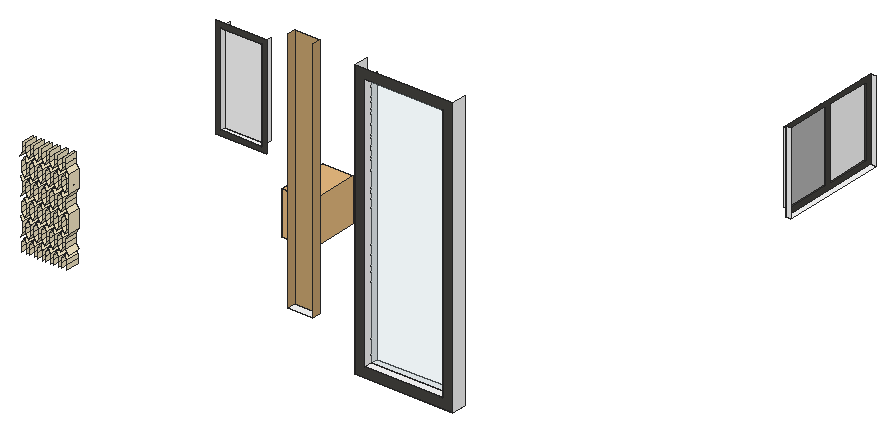
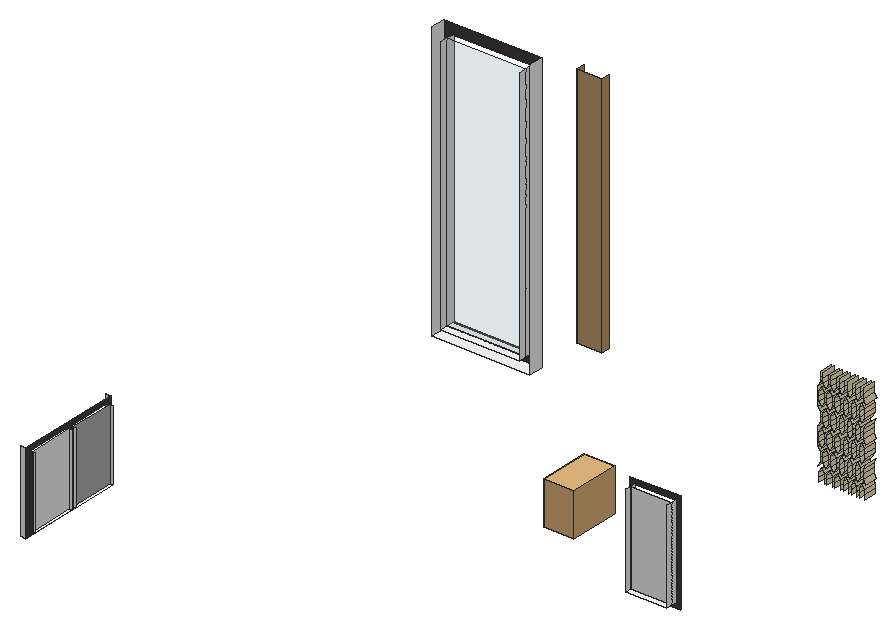
# SketchUp Ruby script. Lengths in inches.
U = 1.inch
M = Sketchup.active_model
def pt(a) = Geom::Point3d.new(a.map { |v| v * U })
def face(e, loops, mat)
  f = e.add_face(loops[0].map { |a| pt(a) })
  loops[1..].each { |l| e.add_face(l.map { |a| pt(a) }).erase! }
  f.material = f.back_material = mat if mat
  f
end
# faces: each face lists its corners as indices into pts; further lists are holes
def faces(e, pts, list, mat = nil) = list.each { |f| face(e, (f[0].is_a?(Array) ? f : [f]).map { |l| l.map { |i| pts[i] } }, mat) }
# xy, xz, yz: faces in a plane at the given z, y or x. An outline is a flat list of corners, or four numbers for a rectangle; further outlines are holes
def ring(l) = l.size == 4 ? [[l[0], l[1]], [l[2], l[1]], [l[2], l[3]], [l[0], l[3]]] : l.each_slice(2).to_a
def flat(e, list, mat, &to3) = list.each { |f| face(e, (f[0].is_a?(Array) ? f : [f]).map { |l| ring(l).map { |u, v| to3.(u, v) } }, mat) }
def xy(e, z, list, mat = nil) = flat(e, list, mat) { |x, y| [x, y, z] }
def xz(e, y, list, mat = nil) = flat(e, list, mat) { |x, z| [x, y, z] }
def yz(e, x, list, mat = nil) = flat(e, list, mat) { |y, z| [x, y, z] }
def lines(e, pts, list) = list.each { |a, b| e.add_line(pt(pts[a]), pt(pts[b])) }
# prism: a flat outline (further loops are holes) pulled along v
def prism(e, loops, v, mat = nil)
  f = face(e, loops, mat); d = Geom::Vector3d.new(v.map { |x| x * U })
  f.pushpull(f.normal.samedirection?(d) ? d.length : -d.length)
end
def box(e, o, s, mat = nil) = prism(e, [[o, [o[0] + s[0], o[1], o[2]], [o[0] + s[0], o[1] + s[1], o[2]], [o[0], o[1] + s[1], o[2]]]], [0, 0, s[2]], mat)
def at(x, y, z, deg = 0) = Geom::Transformation.translation(pt([x, y, z])) * Geom::Transformation.rotation(ORIGIN, Z_AXIS, deg.degrees)
def axes(o, x, y, z) = Geom::Transformation.new([*x, 0, *y, 0, *z, 0, *pt(o).to_a, 1])
def part(name) = M.definitions.add(name)
# library, detail: a bought-in or finely detailed component or shape, given as its bounding box
def library(name, o, s) = part(name).tap { |d| box(d.entities, o, s) }
def detail(e, o, s) = box(e.add_group.entities, o, s)
def put(e, d, t, mat = nil) = e.add_instance(d, t).tap { |i| i.material = mat if mat }
def group(e, t, mat = nil) = e.add_group.tap { |g| g.transformation = t; g.material = mat if mat }.entities
root = M.entities
M.materials.add("D01_Frost_White").color = [255, 242, 206]
M.materials.add("Glass_Mirror_01").color = [185, 185, 185]
M.materials.add("Glass_Safety_01").color = [204, 235, 244]
M.materials["Glass_Safety_01"].alpha = 0.25
M.materials.add("M00_Soft_Cloud").color = [255, 255, 255]
M.materials.add("Plywood_08_1K").color = [202, 166, 113]
M.materials.add("Wood_Planks_01_1K").color = [69, 67, 63]
c1 = library("FF_Model_ID8636_1_ruthrocker1",[-22.29,-12.06,-2.32],[42.44,25.59,36.01])
xy(root,142.2252,[[455.5996,116.0568,536.8247,128.0311]],"M00_Soft_Cloud")
xy(root,145.482,[[189.7692,309,223.7462,313.5],[189.7692,313.5,223.7462,318]],"M00_Soft_Cloud")
xy(root,150.2252,[[463.5996,116.0568,528.8247,122.5284],[463.5996,122.5284,528.8247,129]],"M00_Soft_Cloud")
xy(root,156.7042,[[559.3018,433.068,564,521.5592]],"M00_Soft_Cloud")
xy(root,160.7042,[[555,437.068,557.1509,475.3136],[555,479.3136,557.1509,517.5592]],"M00_Soft_Cloud")
xy(root,160.7042,[[557.1509,437.068,559.3018,475.3136],[557.1509,479.3136,559.3018,517.5592]],"Wood_Planks_01_1K")
xy(root,173.8079,[[402.037,112.9098,423.1418,120]],"M00_Soft_Cloud")
xy(root,197.0101,[[189.8495,109.0676,189.8566,119.6039],[196.5404,109.0676,196.5475,119.6039],[209.9258,109.0676,209.9294,119.6039],[216.6168,109.0676,216.6239,119.6039],[223.3077,109.0676,223.3148,119.6039]],"D01_Frost_White")
xy(root,197.0162,[[189.853,109.0676,189.8602,119.6039],[196.544,109.0676,196.5511,119.6039]],"D01_Frost_White")
xz(root,109.0676,[[216.6203,197.004,216.6239,197.0101,216.6168,197.0101,216.6184,197.0073],[209.9276,197.0071,209.9294,197.0101,209.9258,197.0101],[189.8495,197.0101,189.8566,197.0101,189.8547,197.0134,189.853,197.0162,189.8514,197.0134],[189.8566,197.0101,189.8602,197.0162,189.853,197.0162,189.8547,197.0134],[189.8566,197.0101,189.8637,197.0101,189.8602,197.0162],
  [196.5404,197.0101,196.5475,197.0101,196.5511,197.0162,196.544,197.0162],[196.5475,197.0101,196.5547,197.0101,196.5546,197.0102,196.5511,197.0162],[203.2385,197.0101,203.2456,197.0101,203.2437,197.0134,203.242,197.0162,203.2404,197.0134],[209.933,212.0139,209.933,212.02,209.9312,212.0169]],"D01_Frost_White")
xz(root,116.0568,[[[455.5996,142.2252,536.8247,372.3605],[463.5996,150.2252,528.8247,364.3605]]],"Wood_Planks_01_1K")
xz(root,120,[[402.037,173.8079,423.1418,377.6765]],"Plywood_08_1K")
xz(root,122.5284,[[463.5996,150.2252,528.8247,364.3605]],"Glass_Safety_01")
xz(root,309,[[[185.7692,141.482,227.7462,225.934],[189.7692,145.482,223.7462,221.934]]],"Wood_Planks_01_1K")
xz(root,313.5,[[189.7692,145.482,223.7462,221.934]],"M00_Soft_Cloud")
xz(root,433.068,[[559.3018,156.7042,564,224.1287]],"M00_Soft_Cloud")
xz(root,437.068,[[555,160.7042,557.1509,220.1287]],"M00_Soft_Cloud")
xz(root,437.068,[[557.1509,160.7042,559.3018,220.1287]],"Wood_Planks_01_1K")
xz(root,475.3136,[[555,160.7042,557.1509,220.1287]],"M00_Soft_Cloud")
xz(root,475.3136,[[557.1509,160.7042,559.3018,220.1287]],"Wood_Planks_01_1K")
xz(root,479.3136,[[555,160.7042,557.1509,220.1287],[557.1509,160.7042,559.3018,220.1287]],"M00_Soft_Cloud")
xz(root,517.5592,[[555,160.7042,557.1509,220.1287]],"M00_Soft_Cloud")
xz(root,517.5592,[[557.1509,160.7042,559.3018,220.1287]],"Wood_Planks_01_1K")
xz(root,521.5592,[[559.3018,156.7042,564,224.1287]],"M00_Soft_Cloud")
yz(root,184.3035,[[109.0676,200.7656,119.6039,204.515],[109.0676,204.515,119.6039,208.2645]],"D01_Frost_White")
yz(root,184.3107,[[109.0676,140.7747,119.6039,144.5242],[109.0676,144.5242,119.6039,148.2736],[109.0676,170.7702,119.6039,174.5196],[109.0676,174.5196,119.6039,178.269]],"D01_Frost_White")
yz(root,185.3661,[[109.0676,215.7633,119.6039,219.5128],[109.0676,219.5128,119.6039,223.2622]],"D01_Frost_White")
yz(root,185.3733,[[109.0676,155.7725,119.6039,159.5219],[109.0676,159.5219,119.6039,163.2713],[109.0676,185.7679,119.6039,189.5173],[109.0676,189.5173,119.6039,193.2668]],"D01_Frost_White")
yz(root,187.649,[[109.0676,215.7633,119.6039,219.5128],[109.0676,219.5128,119.6039,223.2622]],"D01_Frost_White")
yz(root,187.6561,[[109.0676,155.7725,119.6039,159.5219],[109.0676,159.5219,119.6039,163.2713],[109.0676,185.7679,119.6039,189.5173],[109.0676,189.5173,119.6039,193.2668]],"D01_Frost_White")
yz(root,188.7116,[[109.0676,200.7656,119.6039,204.515],[109.0676,204.515,119.6039,208.2645]],"D01_Frost_White")
yz(root,188.7188,[[109.0676,140.7747,119.6039,144.5242],[109.0676,144.5242,119.6039,148.2736],[109.0676,170.7702,119.6039,174.5196],[109.0676,174.5196,119.6039,178.269]],"D01_Frost_White")
yz(root,189.7692,[[309,145.482,313.5,221.934],[313.5,145.482,318,221.934]],"M00_Soft_Cloud")
yz(root,190.9945,[[109.0676,200.7656,119.6039,204.515],[109.0676,204.515,119.6039,208.2645]],"D01_Frost_White")
yz(root,191.0016,[[109.0676,140.7747,119.6039,144.5242],[109.0676,144.5242,119.6039,148.2736],[109.0676,170.7702,119.6039,174.5196],[109.0676,174.5196,119.6039,178.269]],"D01_Frost_White")
yz(root,192.0571,[[109.0676,215.7633,119.6039,219.5128],[109.0676,219.5128,119.6039,223.2622]],"D01_Frost_White")
yz(root,192.0642,[[109.0676,155.7725,119.6039,159.5219],[109.0676,159.5219,119.6039,163.2713],[109.0676,185.7679,119.6039,189.5173],[109.0676,189.5173,119.6039,193.2668]],"D01_Frost_White")
yz(root,194.3399,[[109.0676,215.7633,119.6039,219.5128],[109.0676,219.5128,119.6039,223.2622]],"D01_Frost_White")
yz(root,194.3471,[[109.0676,155.7725,119.6039,159.5219],[109.0676,159.5219,119.6039,163.2713],[109.0676,185.7679,119.6039,189.5173],[109.0676,189.5173,119.6039,193.2668]],"D01_Frost_White")
yz(root,195.4025,[[109.0676,200.7656,119.6039,204.515],[109.0676,204.515,119.6039,208.2645]],"D01_Frost_White")
yz(root,195.4097,[[109.0676,140.7747,119.6039,144.5242],[109.0676,144.5242,119.6039,148.2736],[109.0676,170.7702,119.6039,174.5196],[109.0676,174.5196,119.6039,178.269]],"D01_Frost_White")
yz(root,197.6925,[[109.0676,140.7747,119.6039,144.5242],[109.0676,144.5242,119.6039,148.2736],[109.0676,170.7702,119.6039,174.5196],[109.0676,174.5196,119.6039,178.269],[109.0676,200.7656,119.6039,204.515],
  [109.0676,204.515,119.6039,208.2645]],"D01_Frost_White")
yz(root,198.748,[[109.0676,215.7633,119.6039,223.2622]],"D01_Frost_White")
yz(root,198.7552,[[109.0676,155.7725,119.6039,159.5219],[109.0676,159.5219,119.6039,163.2713],[109.0676,185.7679,119.6039,189.5173],[109.0676,189.5173,119.6039,193.2668]],"D01_Frost_White")
yz(root,201.038,[[109.0676,155.7725,119.6039,159.5219],[109.0676,159.5219,119.6039,163.2713],[109.0676,185.7679,119.6039,189.5173],[109.0676,189.5173,119.6039,193.2668],[109.0676,215.7633,119.6039,219.5128],
  [109.0676,219.5128,119.6039,223.2622]],"D01_Frost_White")
yz(root,202.1006,[[109.0676,140.7747,119.6039,144.5242],[109.0676,144.5242,119.6039,148.2736],[109.0676,170.7702,119.6039,174.5196],[109.0676,174.5196,119.6039,178.269],[109.0676,200.7656,119.6039,204.515],
  [109.0676,204.515,119.6039,208.2645]],"D01_Frost_White")
yz(root,204.3835,[[109.0676,140.7747,119.6039,144.5242],[109.0676,144.5242,119.6039,148.2736],[109.0676,170.7702,119.6039,174.5196],[109.0676,174.5196,119.6039,178.269],[109.0676,200.7656,119.6039,204.515],
  [109.0676,204.515,119.6039,208.2645]],"D01_Frost_White")
yz(root,205.4461,[[109.0676,155.7725,119.6039,159.5219],[109.0676,159.5219,119.6039,163.2713],[109.0676,185.7679,119.6039,189.5173],[109.0676,189.5173,119.6039,193.2668],[109.0676,215.7633,119.6039,219.5128],
  [109.0676,219.5128,119.6039,223.2622]],"D01_Frost_White")
yz(root,207.7289,[[109.0676,155.7725,119.6039,159.5219],[109.0676,159.5219,119.6039,163.2713],[109.0676,185.7679,119.6039,189.5173],[109.0676,189.5173,119.6039,193.2668],[109.0676,215.7633,119.6039,219.5128],
  [109.0676,219.5128,119.6039,223.2622]],"D01_Frost_White")
yz(root,208.7916,[[109.0676,140.7747,119.6039,144.5242],[109.0676,144.5242,119.6039,148.2736],[109.0676,170.7702,119.6039,174.5196],[109.0676,174.5196,119.6039,178.269],[109.0676,200.7656,119.6039,204.515],
  [109.0676,204.515,119.6039,208.2645]],"D01_Frost_White")
yz(root,209.933,[[109.0676,152.0169,119.6039,152.023],[109.0676,167.0147,119.6039,167.0207],[109.0676,182.0124,119.6039,182.0185],[109.0676,197.0101,119.6039,197.0162],[109.0676,212.0139,119.6039,212.02]],"D01_Frost_White")
yz(root,211.0673,[[109.0676,200.7595,119.6039,204.509],[109.0676,204.509,119.6039,208.2584]],"D01_Frost_White")
yz(root,211.0744,[[109.0676,140.7687,119.6039,144.5181],[109.0676,144.5181,119.6039,148.2675],[109.0676,170.7641,119.6039,174.5135],[109.0676,174.5135,119.6039,178.263]],"D01_Frost_White")
yz(root,212.1299,[[109.0676,215.7573,119.6039,219.5067],[109.0676,219.5067,119.6039,223.2561]],"D01_Frost_White")
yz(root,212.137,[[109.0676,155.7664,119.6039,159.5158],[109.0676,159.5158,119.6039,163.2652],[109.0676,185.7618,119.6039,189.5113],[109.0676,189.5113,119.6039,193.2607]],"D01_Frost_White")
yz(root,214.4127,[[109.0676,215.7573,119.6039,219.5067],[109.0676,219.5067,119.6039,223.2561]],"D01_Frost_White")
yz(root,214.4199,[[109.0676,155.7664,119.6039,159.5158],[109.0676,159.5158,119.6039,163.2652],[109.0676,185.7618,119.6039,189.5113],[109.0676,189.5113,119.6039,193.2607]],"D01_Frost_White")
yz(root,215.4754,[[109.0676,200.7595,119.6039,204.509],[109.0676,204.509,119.6039,208.2584]],"D01_Frost_White")
yz(root,215.4825,[[109.0676,140.7687,119.6039,144.5181],[109.0676,144.5181,119.6039,148.2675],[109.0676,170.7641,119.6039,174.5135],[109.0676,174.5135,119.6039,178.263]],"D01_Frost_White")
yz(root,217.7582,[[109.0676,200.7595,119.6039,204.509],[109.0676,204.509,119.6039,208.2584]],"D01_Frost_White")
yz(root,217.7653,[[109.0676,140.7687,119.6039,144.5181],[109.0676,144.5181,119.6039,148.2675],[109.0676,170.7641,119.6039,174.5135],[109.0676,174.5135,119.6039,178.263]],"D01_Frost_White")
yz(root,218.8208,[[109.0676,215.7573,119.6039,219.5067],[109.0676,219.5067,119.6039,223.2561]],"D01_Frost_White")
yz(root,218.828,[[109.0676,155.7664,119.6039,159.5158],[109.0676,159.5158,119.6039,163.2652],[109.0676,185.7618,119.6039,189.5113],[109.0676,189.5113,119.6039,193.2607]],"D01_Frost_White")
yz(root,221.1037,[[109.0676,215.7573,119.6039,219.5067],[109.0676,219.5067,119.6039,223.2561]],"D01_Frost_White")
yz(root,221.1108,[[109.0676,155.7664,119.6039,159.5158],[109.0676,159.5158,119.6039,163.2652],[109.0676,185.7618,119.6039,189.5113],[109.0676,189.5113,119.6039,193.2607]],"D01_Frost_White")
yz(root,222.1663,[[109.0676,200.7595,119.6039,204.509],[109.0676,204.509,119.6039,208.2584]],"D01_Frost_White")
yz(root,222.1734,[[109.0676,140.7687,119.6039,144.5181],[109.0676,144.5181,119.6039,148.2675],[109.0676,170.7641,119.6039,174.5135],[109.0676,174.5135,119.6039,178.263]],"D01_Frost_White")
yz(root,223.3077,[[109.0676,197.0101,119.6039,212.0078]],"D01_Frost_White")
yz(root,223.3148,[[109.0676,167.0147,119.6039,182.0124]],"D01_Frost_White")
yz(root,223.7462,[[309,145.482,313.5,221.934],[313.5,145.482,318,221.934]],"M00_Soft_Cloud")
yz(root,402.037,[[112.9098,173.8079,120,377.6765]],"Plywood_08_1K")
yz(root,423.1418,[[112.9098,173.8079,120,377.6765]],"Plywood_08_1K")
yz(root,455.5996,[[116.0568,142.2252,128.0311,372.3605]],"M00_Soft_Cloud")
yz(root,463.5996,[[116.0568,150.2252,122.5284,364.3605],[122.5284,150.2252,129,364.3605]],"M00_Soft_Cloud")
yz(root,528.8247,[[116.0568,150.2252,122.5284,364.3605],[122.5284,150.2252,129,364.3605]],"M00_Soft_Cloud")
yz(root,536.8247,[[116.0568,142.2252,128.0311,372.3605]],"M00_Soft_Cloud")
yz(root,557.1509,[[437.068,160.7042,475.3136,220.1287]],"Glass_Mirror_01")
yz(root,557.1509,[[479.3136,160.7042,517.5592,220.1287]],"M00_Soft_Cloud")
yz(root,559.3018,[[[433.068,156.7042,521.5592,224.1287],[437.068,160.7042,475.3136,220.1287],[479.3136,160.7042,517.5592,220.1287]]],"Wood_Planks_01_1K")
p = [[184.3107,109.0676,148.2736],[186.5147,109.0676,152.023],[186.5147,119.6039,152.023],[184.3107,119.6039,148.2736],[188.7188,109.0676,148.2736],[188.7188,119.6039,148.2736],
  [191.0016,109.0676,148.2736],[193.2056,109.0676,152.023],[193.2056,119.6039,152.023],[191.0016,119.6039,148.2736],[195.4097,109.0676,148.2736],[195.4097,119.6039,148.2736],
  [197.6925,109.0676,148.2736],[199.8966,109.0676,152.023],[199.8966,119.6039,152.023],[197.6925,119.6039,148.2736],[202.1006,109.0676,148.2736],[202.1006,119.6039,148.2736],
  [204.3835,109.0676,148.2736],[206.5875,109.0676,152.023],[206.5875,119.6039,152.023],[204.3835,119.6039,148.2736],[208.7916,109.0676,148.2736],[208.7916,119.6039,148.2736],
  [211.0744,109.0676,148.2675],[213.2784,109.0676,152.0169],[213.2784,119.6039,152.0169],[211.0744,119.6039,148.2675],[215.4825,109.0676,148.2675],[215.4825,119.6039,148.2675],
  [217.7653,109.0676,148.2675],[219.9694,109.0676,152.0169],[219.9694,119.6039,152.0169],[217.7653,119.6039,148.2675],[222.1734,109.0676,148.2675],[222.1734,119.6039,148.2675],
  [185.3733,109.0676,155.7725],[183.1692,109.0676,152.023],[183.1692,119.6039,152.023],[185.3733,119.6039,155.7725],[189.8602,109.0676,152.023],[187.6561,109.0676,155.7725],
  [187.6561,119.6039,155.7725],[189.8602,119.6039,152.023],[192.0642,109.0676,155.7725],[192.0642,119.6039,155.7725],[196.5511,109.0676,152.023],[194.3471,109.0676,155.7725],
  [194.3471,119.6039,155.7725],[196.5511,119.6039,152.023],[198.7552,109.0676,155.7725],[198.7552,119.6039,155.7725],[203.242,109.0676,152.023],[201.038,109.0676,155.7725],
  [201.038,119.6039,155.7725],[203.242,119.6039,152.023],[205.4461,109.0676,155.7725],[205.4461,119.6039,155.7725],[209.933,109.0676,152.023],[207.7289,109.0676,155.7725],
  [207.7289,119.6039,155.7725],[209.933,119.6039,152.023],[212.137,109.0676,155.7664],[209.933,109.0676,152.0169],[209.933,119.6039,152.0169],[212.137,119.6039,155.7664],
  [216.6239,109.0676,152.0169],[214.4199,109.0676,155.7664],[214.4199,119.6039,155.7664],[216.6239,119.6039,152.0169],[218.828,109.0676,155.7664],[218.828,119.6039,155.7664],
  [223.3148,109.0676,152.0169],[221.1108,109.0676,155.7664],[221.1108,119.6039,155.7664],[223.3148,119.6039,152.0169],[183.1692,109.0676,167.0207],[185.3733,109.0676,163.2713],
  [185.3733,119.6039,163.2713],[183.1692,119.6039,167.0207],[187.6561,109.0676,163.2713],[189.8602,109.0676,167.0207],[189.8602,119.6039,167.0207],[187.6561,119.6039,163.2713],
  [192.0642,109.0676,163.2713],[192.0642,119.6039,163.2713],[194.3471,109.0676,163.2713],[196.5511,109.0676,167.0207],[196.5511,119.6039,167.0207],[194.3471,119.6039,163.2713],
  [198.7552,109.0676,163.2713],[198.7552,119.6039,163.2713],[201.038,109.0676,163.2713],[203.242,109.0676,167.0207],[203.242,119.6039,167.0207],[201.038,119.6039,163.2713],
  [205.4461,109.0676,163.2713],[205.4461,119.6039,163.2713],[207.7289,109.0676,163.2713],[209.933,109.0676,167.0207],[209.933,119.6039,167.0207],[207.7289,119.6039,163.2713],
  [209.933,109.0676,167.0147],[212.137,109.0676,163.2652],[212.137,119.6039,163.2652],[209.933,119.6039,167.0147],[214.4199,109.0676,163.2652],[216.6239,109.0676,167.0147],
  [216.6239,119.6039,167.0147],[214.4199,119.6039,163.2652],[218.828,109.0676,163.2652],[218.828,119.6039,163.2652],[221.1108,109.0676,163.2652],[223.3148,109.0676,167.0147],
  [223.3148,119.6039,167.0147],[221.1108,119.6039,163.2652],[186.5147,109.0676,167.0207],[184.3107,109.0676,170.7702],[184.3107,119.6039,170.7702],[186.5147,119.6039,167.0207],
  [188.7188,109.0676,170.7702],[188.7188,119.6039,170.7702],[193.2056,109.0676,167.0207],[191.0016,109.0676,170.7702],[191.0016,119.6039,170.7702],[193.2056,119.6039,167.0207],
  [195.4097,109.0676,170.7702],[195.4097,119.6039,170.7702],[199.8966,109.0676,167.0207],[197.6925,109.0676,170.7702],[197.6925,119.6039,170.7702],[199.8966,119.6039,167.0207],
  [202.1006,109.0676,170.7702],[202.1006,119.6039,170.7702],[206.5875,109.0676,167.0207],[204.3835,109.0676,170.7702],[204.3835,119.6039,170.7702],[206.5875,119.6039,167.0207],
  [208.7916,109.0676,170.7702],[208.7916,119.6039,170.7702],[213.2784,109.0676,167.0147],[211.0744,109.0676,170.7641],[211.0744,119.6039,170.7641],[213.2784,119.6039,167.0147],
  [215.4825,109.0676,170.7641],[215.4825,119.6039,170.7641],[219.9694,109.0676,167.0147],[217.7653,109.0676,170.7641],[217.7653,119.6039,170.7641],[219.9694,119.6039,167.0147],
  [222.1734,109.0676,170.7641],[222.1734,119.6039,170.7641],[184.3107,109.0676,178.269],[186.5147,109.0676,182.0185],[186.5147,119.6039,182.0185],[184.3107,119.6039,178.269],
  [188.7188,109.0676,178.269],[188.7188,119.6039,178.269],[191.0016,109.0676,178.269],[193.2056,109.0676,182.0185],[193.2056,119.6039,182.0185],[191.0016,119.6039,178.269],
  [195.4097,109.0676,178.269],[195.4097,119.6039,178.269],[197.6925,109.0676,178.269],[199.8966,109.0676,182.0185],[199.8966,119.6039,182.0185],[197.6925,119.6039,178.269],
  [202.1006,109.0676,178.269],[202.1006,119.6039,178.269],[204.3835,109.0676,178.269],[206.5875,109.0676,182.0185],[206.5875,119.6039,182.0185],[204.3835,119.6039,178.269],
  [208.7916,109.0676,178.269],[208.7916,119.6039,178.269],[211.0744,109.0676,178.263],[213.2784,109.0676,182.0124],[213.2784,119.6039,182.0124],[211.0744,119.6039,178.263],
  [215.4825,109.0676,178.263],[215.4825,119.6039,178.263],[217.7653,109.0676,178.263],[219.9694,109.0676,182.0124],[219.9694,119.6039,182.0124],[217.7653,119.6039,178.263],
  [222.1734,109.0676,178.263],[222.1734,119.6039,178.263],[185.3733,109.0676,185.7679],[183.1692,109.0676,182.0185],[183.1692,119.6039,182.0185],[185.3733,119.6039,185.7679],
  [189.8602,109.0676,182.0185],[187.6561,109.0676,185.7679],[187.6561,119.6039,185.7679],[189.8602,119.6039,182.0185],[192.0642,109.0676,185.7679],[192.0642,119.6039,185.7679],
  [196.5511,109.0676,182.0185],[194.3471,109.0676,185.7679],[194.3471,119.6039,185.7679],[196.5511,119.6039,182.0185],[198.7552,109.0676,185.7679],[198.7552,119.6039,185.7679],
  [203.242,109.0676,182.0185],[201.038,109.0676,185.7679],[201.038,119.6039,185.7679],[203.242,119.6039,182.0185],[205.4461,109.0676,185.7679],[205.4461,119.6039,185.7679],
  [209.933,109.0676,182.0185],[207.7289,109.0676,185.7679],[207.7289,119.6039,185.7679],[209.933,119.6039,182.0185],[212.137,109.0676,185.7618],[209.933,109.0676,182.0124],
  [209.933,119.6039,182.0124],[212.137,119.6039,185.7618],[216.6239,109.0676,182.0124],[214.4199,109.0676,185.7618],[214.4199,119.6039,185.7618],[216.6239,119.6039,182.0124],
  [218.828,109.0676,185.7618],[218.828,119.6039,185.7618],[223.3148,109.0676,182.0124],[221.1108,109.0676,185.7618],[221.1108,119.6039,185.7618],[223.3148,119.6039,182.0124],
  [183.1728,109.0676,197.0101],[185.3733,109.0676,193.2668],[185.3733,119.6039,193.2668],[183.1728,119.6039,197.0101],[187.6561,109.0676,193.2668],[189.8566,109.0676,197.0101],
  [189.8566,119.6039,197.0101],[187.6561,119.6039,193.2668],[189.8637,109.0676,197.0101],[192.0642,109.0676,193.2668],[192.0642,119.6039,193.2668],[189.8637,119.6039,197.0101],
  [194.3471,109.0676,193.2668],[196.5475,109.0676,197.0101],[196.5475,119.6039,197.0101],[194.3471,119.6039,193.2668],[196.5547,109.0676,197.0101],[198.7552,109.0676,193.2668],
  [198.7552,119.6039,193.2668],[196.5547,119.6039,197.0101],[201.038,109.0676,193.2668],[203.2385,109.0676,197.0101],[203.2385,119.6039,197.0101],[201.038,119.6039,193.2668],
  [203.2456,109.0676,197.0101],[205.4461,109.0676,193.2668],[205.4461,119.6039,193.2668],[203.2456,119.6039,197.0101],[207.7289,109.0676,193.2668],[209.9276,109.0676,197.0071],
  [209.9276,119.6039,197.0071],[207.7289,119.6039,193.2668],[209.933,109.0676,197.0101],[212.137,109.0676,193.2607],[212.137,119.6039,193.2607],[209.933,119.6039,197.0101],
  [214.4199,109.0676,193.2607],[216.6203,109.0676,197.004],[216.6203,119.6039,197.004],[214.4199,119.6039,193.2607],[216.6239,109.0676,197.0101],[218.828,109.0676,193.2607],
  [218.828,119.6039,193.2607],[216.6239,119.6039,197.0101],[221.1108,109.0676,193.2607],[223.3148,109.0676,197.0101],[223.3148,119.6039,197.0101],[221.1108,119.6039,193.2607],
  [186.5076,109.0676,197.0162],[184.3035,109.0676,200.7656],[184.3035,119.6039,200.7656],[186.5076,119.6039,197.0162],[188.7116,109.0676,200.7656],[188.7116,119.6039,200.7656],
  [189.8495,109.0676,197.0101],[189.8514,109.0676,197.0134],[189.8514,119.6039,197.0134],[189.8495,119.6039,197.0101],[189.853,109.0676,197.0162],[189.853,119.6039,197.0162],
  [189.8602,109.0676,197.0162],[189.8602,119.6039,197.0162],[193.1985,109.0676,197.0162],[190.9945,109.0676,200.7656],[190.9945,119.6039,200.7656],[193.1985,119.6039,197.0162],
  [195.4025,109.0676,200.7656],[195.4025,119.6039,200.7656],[196.5404,109.0676,197.0101],[196.544,109.0676,197.0162],[196.544,119.6039,197.0162],[196.5404,119.6039,197.0101],
  [196.5511,109.0676,197.0162],[196.5546,109.0676,197.0102],[196.5546,119.6039,197.0102],[196.5511,119.6039,197.0162],[199.8966,109.0676,197.0162],[197.6925,109.0676,200.7656],
  [197.6925,119.6039,200.7656],[199.8966,119.6039,197.0162],[202.1006,109.0676,200.7656],[202.1006,119.6039,200.7656],[203.2404,109.0676,197.0134],[203.2404,119.6039,197.0134],
  [203.242,109.0676,197.0162],[203.242,119.6039,197.0162],[203.2437,109.0676,197.0134],[203.2437,119.6039,197.0134],[206.5875,109.0676,197.0162],[204.3835,109.0676,200.7656],
  [204.3835,119.6039,200.7656],[206.5875,119.6039,197.0162],[208.7916,109.0676,200.7656],[208.7916,119.6039,200.7656],[209.9258,109.0676,197.0101],[209.9258,119.6039,197.0101],
  [209.9294,109.0676,197.0101],[209.933,109.0676,197.0162],[209.933,119.6039,197.0162],[209.9294,119.6039,197.0101],[213.2713,109.0676,197.0101],[211.0673,109.0676,200.7595],
  [211.0673,119.6039,200.7595],[213.2713,119.6039,197.0101],[215.4754,109.0676,200.7595],[215.4754,119.6039,200.7595],[216.6184,109.0676,197.0073],[216.6168,109.0676,197.0101],
  [216.6168,119.6039,197.0101],[216.6184,119.6039,197.0073],[219.9622,109.0676,197.0101],[217.7582,109.0676,200.7595],[217.7582,119.6039,200.7595],[219.9622,119.6039,197.0101],
  [222.1663,109.0676,200.7595],[222.1663,119.6039,200.7595],[184.3035,109.0676,208.2645],[186.5076,109.0676,212.0139],[186.5076,119.6039,212.0139],[184.3035,119.6039,208.2645],
  [188.7116,109.0676,208.2645],[188.7116,119.6039,208.2645],[190.9945,109.0676,208.2645],[193.1985,109.0676,212.0139],[193.1985,119.6039,212.0139],[190.9945,119.6039,208.2645],
  [195.4025,109.0676,208.2645],[195.4025,119.6039,208.2645],[197.6925,109.0676,208.2645],[199.8966,109.0676,212.0139],[199.8966,119.6039,212.0139],[197.6925,119.6039,208.2645],
  [202.1006,109.0676,208.2645],[202.1006,119.6039,208.2645],[204.3835,109.0676,208.2645],[206.5875,109.0676,212.0139],[206.5875,119.6039,212.0139],[204.3835,119.6039,208.2645],
  [208.7916,109.0676,208.2645],[208.7916,119.6039,208.2645],[211.0673,109.0676,208.2584],[213.2713,109.0676,212.0078],[213.2713,119.6039,212.0078],[211.0673,119.6039,208.2584],
  [215.4754,109.0676,208.2584],[215.4754,119.6039,208.2584],[217.7582,109.0676,208.2584],[219.9622,109.0676,212.0078],[219.9622,119.6039,212.0078],[217.7582,119.6039,208.2584],
  [222.1663,109.0676,208.2584],[222.1663,119.6039,208.2584],[185.3661,109.0676,215.7633],[183.1675,109.0676,212.023],[183.1675,119.6039,212.023],[185.3661,119.6039,215.7633],
  [189.853,109.0676,212.0139],[187.649,109.0676,215.7633],[187.649,119.6039,215.7633],[189.853,119.6039,212.0139],[192.0571,109.0676,215.7633],[192.0571,119.6039,215.7633],
  [196.544,109.0676,212.0139],[194.3399,109.0676,215.7633],[194.3399,119.6039,215.7633],[196.544,119.6039,212.0139],[198.748,109.0676,215.7633],[198.748,119.6039,215.7633],
  [203.242,109.0676,212.0139],[201.038,109.0676,215.7633],[201.038,119.6039,215.7633],[203.242,119.6039,212.0139],[205.4461,109.0676,215.7633],[205.4461,119.6039,215.7633],
  [209.9312,109.0676,212.0169],[207.7289,109.0676,215.7633],[207.7289,119.6039,215.7633],[209.9312,119.6039,212.0169],[209.933,109.0676,212.0139],[209.933,119.6039,212.0139],
  [212.1299,109.0676,215.7573],[209.933,109.0676,212.02],[209.933,119.6039,212.02],[212.1299,119.6039,215.7573],[216.6168,109.0676,212.0078],[214.4127,109.0676,215.7573],
  [214.4127,119.6039,215.7573],[216.6168,119.6039,212.0078],[218.8208,109.0676,215.7573],[218.8208,119.6039,215.7573],[223.3077,109.0676,212.0078],[221.1037,109.0676,215.7573],
  [221.1037,119.6039,215.7573],[223.3077,119.6039,212.0078],[209.9276,109.0676,212.0109],[223.3041,109.0676,197.004],[223.3077,109.0676,197.0101],[209.9294,109.0676,197.0041],
  [209.9258,109.0676,212.0078],[209.9294,109.0676,197.004],[216.6151,109.0676,197.0074],[216.6132,109.0676,197.004]]
faces(root,p,[[0,1,2,3],[1,4,5,2],[6,7,8,9],[7,10,11,8],[12,13,14,15],[13,16,17,14],[18,19,20,21],[19,22,23,20],
  [24,25,26,27],[25,28,29,26],[30,31,32,33],[31,34,35,32],[36,37,38,39],[40,41,42,43],[44,40,43,45],[46,47,48,49],
  [50,46,49,51],[52,53,54,55],[56,52,55,57],[58,59,60,61],[62,63,64,65],[66,67,68,69],[70,66,69,71],[72,73,74,75],
  [76,77,78,79],[80,81,82,83],[81,84,85,82],[86,87,88,89],[87,90,91,88],[92,93,94,95],[93,96,97,94],[98,99,100,101],
  [102,103,104,105],[106,107,108,109],[107,110,111,108],[112,113,114,115],[116,117,118,119],[120,116,119,121],[122,123,124,125],[126,122,125,127],
  [128,129,130,131],[132,128,131,133],[134,135,136,137],[138,134,137,139],[140,141,142,143],[144,140,143,145],[146,147,148,149],[150,146,149,151],
  [152,153,154,155],[153,156,157,154],[158,159,160,161],[159,162,163,160],[164,165,166,167],[165,168,169,166],[170,171,172,173],[171,174,175,172],
  [176,177,178,179],[177,180,181,178],[182,183,184,185],[183,186,187,184],[188,189,190,191],[192,193,194,195],[196,192,195,197],[198,199,200,201],
  [202,198,201,203],[204,205,206,207],[208,204,207,209],[210,211,212,213],[214,215,216,217],[218,219,220,221],[222,218,221,223],[224,225,226,227],
  [228,229,230,231],[232,233,234,235],[236,237,238,239],[240,241,242,243],[244,245,246,247],[248,249,250,251],[252,253,254,255],[256,257,258,259],
  [260,261,262,263],[264,265,266,267],[268,269,270,271],[272,273,274,275],[276,277,278,279],[280,276,279,281],[282,283,284,285],[283,286,287,284],
  [288,236,239,289],[290,291,292,293],[294,290,293,295],[296,297,298,299],[300,301,302,303],[301,244,247,302],[304,305,306,307],[308,304,307,309],
  [249,310,311,250],[310,312,313,311],[312,314,315,313],[314,252,255,315],[316,317,318,319],[320,316,319,321],[257,322,323,258],[324,325,326,327],
  [328,329,330,331],[332,328,331,333],[334,335,336,337],[265,334,337,266],[338,339,340,341],[342,338,341,343],[344,345,346,347],[345,348,349,346],
  [350,351,352,353],[351,354,355,352],[356,357,358,359],[357,360,361,358],[362,363,364,365],[363,366,367,364],[368,369,370,371],[369,372,373,370],
  [374,375,376,377],[375,378,379,376],[380,381,382,383],[384,385,386,387],[388,384,387,389],[390,391,392,393],[394,390,393,395],[396,397,398,399],
  [400,396,399,401],[402,403,404,405],[406,402,405,407],[408,409,410,411],[412,413,414,415],[416,412,415,417],[418,419,420,421]],"D01_Frost_White")
lines(root,p,[[402,422],[423,424],[257,425],[422,426],[425,427],[428,335],[429,428]])
put(root,c1,at(313.07,253.1,141.02,-90))
